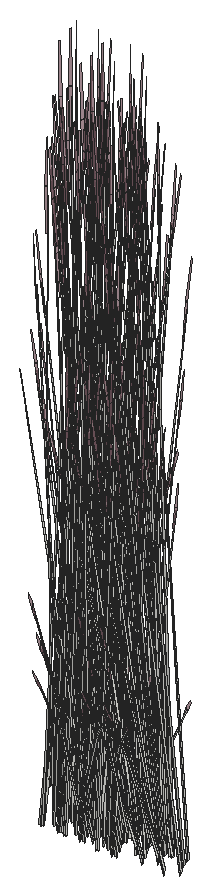
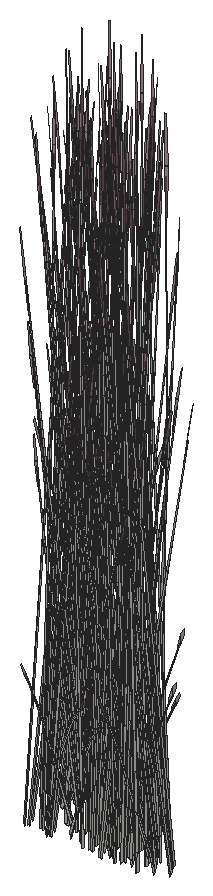
# SketchUp Ruby script. Lengths in inches.
U = 1.inch
M = Sketchup.active_model
def pt(a) = Geom::Point3d.new(a.map { |v| v * U })
def face(e, loops, mat)
  f = e.add_face(loops[0].map { |a| pt(a) })
  loops[1..].each { |l| e.add_face(l.map { |a| pt(a) }).erase! }
  f.material = f.back_material = mat if mat
  f
end
# faces: each face lists its corners as indices into pts; further lists are holes
def faces(e, pts, list, mat = nil) = list.each { |f| face(e, (f[0].is_a?(Array) ? f : [f]).map { |l| l.map { |i| pts[i] } }, mat) }
# xy, xz, yz: faces in a plane at the given z, y or x. An outline is a flat list of corners, or four numbers for a rectangle; further outlines are holes
def ring(l) = l.size == 4 ? [[l[0], l[1]], [l[2], l[1]], [l[2], l[3]], [l[0], l[3]]] : l.each_slice(2).to_a
def flat(e, list, mat, &to3) = list.each { |f| face(e, (f[0].is_a?(Array) ? f : [f]).map { |l| ring(l).map { |u, v| to3.(u, v) } }, mat) }
def xy(e, z, list, mat = nil) = flat(e, list, mat) { |x, y| [x, y, z] }
def xz(e, y, list, mat = nil) = flat(e, list, mat) { |x, z| [x, y, z] }
def yz(e, x, list, mat = nil) = flat(e, list, mat) { |y, z| [x, y, z] }
def lines(e, pts, list) = list.each { |a, b| e.add_line(pt(pts[a]), pt(pts[b])) }
# prism: a flat outline (further loops are holes) pulled along v
def prism(e, loops, v, mat = nil)
  f = face(e, loops, mat); d = Geom::Vector3d.new(v.map { |x| x * U })
  f.pushpull(f.normal.samedirection?(d) ? d.length : -d.length)
end
def box(e, o, s, mat = nil) = prism(e, [[o, [o[0] + s[0], o[1], o[2]], [o[0] + s[0], o[1] + s[1], o[2]], [o[0], o[1] + s[1], o[2]]]], [0, 0, s[2]], mat)
def at(x, y, z, deg = 0) = Geom::Transformation.translation(pt([x, y, z])) * Geom::Transformation.rotation(ORIGIN, Z_AXIS, deg.degrees)
def axes(o, x, y, z) = Geom::Transformation.new([*x, 0, *y, 0, *z, 0, *pt(o).to_a, 1])
def part(name) = M.definitions.add(name)
# library, detail: a bought-in or finely detailed component or shape, given as its bounding box
def library(name, o, s) = part(name).tap { |d| box(d.entities, o, s) }
def detail(e, o, s) = box(e.add_group.entities, o, s)
def put(e, d, t, mat = nil) = e.add_instance(d, t).tap { |i| i.material = mat if mat }
def group(e, t, mat = nil) = e.add_group.tap { |g| g.transformation = t; g.material = mat if mat }.entities
root = M.entities
M.materials.add("LightPink_Translucent").color = [144, 107, 117]
M.materials["LightPink_Translucent"].alpha = 0.75
c1 = part("blade")
p = [[2.15,0.21,22],[0,0.17,0],[0.09,0.45,0],[2.18,0.31,22],[2.29,0.31,22],[0.38,0.45,0],
  [2.48,0.24,33],[2.49,0.24,33],[2.48,0.22,33]]
faces(c1.entities,p,[[0,1,2,3],[4,5,2,3],[6,3,4,7],[8,0,3,6]])
c2 = part("seeds")
p = [[0.3,-0.1,1.38],[-0.01,-0.03,1.59],[-0.01,-0.03,0.03],[0.14,-0.07,-0.07],[0.29,-0.03,3],[0.15,0.01,3.11]]
faces(c2.entities,p,[[0,1,2,3],[1,0,4,5]],"LightPink_Translucent")
c3 = part("blade with seeds")
put(c3.entities,c1,at(0,0,0))
put(c3.entities,c2,axes([2.4,0.25,30.99],[1.5799,-0.05474,1.17369],[-0.12525,1.92788,0.29478],[-0.07173,-0.02425,1.56792]))
put(root,c3,axes([347.7,353.87,622.68],[-0.25628,0.30892,-0.51099],[-0.22444,-0.32634,-0.3958],[-0.13021,-0.047,0.97773]))
put(root,c3,axes([347.29,354.76,619.49],[0.00895,0.0735,1.76342],[-0.18044,0.38382,-0.26939],[-0.12817,-0.01935,0.30037]))
put(root,c3,axes([343.2,353.8,620.02],[0.33032,0.23318,-0.49651],[-0.19744,0.41812,0],[0.07523,0.05311,1.57504]))
put(root,c3,axes([344.44,355.23,620.21],[0.39487,0,0],[0,0.48281,0],[0,0,1.78407]))
put(root,c3,axes([347.34,353.01,622.71],[0.02617,0.04654,1.77383],[-0.12614,0.41836,-0.16761],[-0.12775,0.00303,0.31391]))
put(root,c3,axes([344.0625,354.7,620.72],[-0.21202,-0.39143,0.44739],[0.32115,-0.27564,-0.21531],[0.06861,0.04843,1.43643]))
put(root,c3,axes([344.66,354.73,620.03],[0.24637,-0.29097,-0.30978],[0.24637,0.29097,0.30978],[0,-0.09372,1.38974]))
put(root,c3,axes([343.68,354.79,620.67],[-0.04113,-0.53214,-0.29095],[0.42835,-0.03218,-0.50002],[0.07543,-0.07088,1.59708]))
put(root,c3,axes([345.68,355.49,620.36],[0.44609,0.09826,0.45755],[-0.09078,0.55493,0.17955],[-0.06519,-0.05359,1.58856]))
put(root,c3,axes([343.41,355.48,623.05],[-0.29332,-0.1301,0.35414],[0.08555,-0.37955,-0.4572],[0.11809,-0.0348,0.87481]))
put(root,c3,axes([347.32,354.55,622.73],[0.09971,-0.42522,0.48003],[0.32782,0.1454,0.3958],[-0.12892,0.02555,0.9933]))
put(root,c3,axes([342.72,354.69,620.06],[0.36714,0.07646,-0.62353],[-0.07747,0.47163,-0.16365],[0.10956,0.05715,1.37633]))
put(root,c3,axes([347.84,353.55,623.03],[-0.0189,0.47427,-0.1216],[-0.35781,-0.01296,-0.67495],[-0.13781,-0.03295,1.02557]))
put(root,c3,axes([345.56,355.39,620.72],[-0.17124,0.42022,0.44739],[-0.35581,-0.20224,-0.21531],[0,-0.09687,1.43643]))
put(root,c3,axes([344.28,354.97,620.26],[-0.21881,-0.29821,-0.06488],[0.23965,-0.27324,-0.29416],[0.0679,-0.01924,0.97024]))
put(root,c3,axes([347.29,354.43,622.73],[-0.12963,-0.31798,0.0643],[0.23638,-0.15564,0.50621],[-0.1042,0.03071,0.77189]))
put(root,c3,axes([343.62,353.61,620.03],[0.32928,0.11539,-0.30978],[-0.08291,0.40636,0.30978],[0.06638,-0.04686,1.38974]))
put(root,c3,axes([343.64,354.51,622.73],[0.2423,0.19613,0.0643],[-0.14107,0.2793,0.50621],[0.07768,-0.0903,0.77189]))
put(root,c3,axes([345.4375,356.37,620.47],[0.37926,-0.12378,0.17642],[0.09365,0.46065,0.35086],[-0.03382,-0.06712,1.60407]))
put(root,c3,axes([347.125,354.28,620.77],[0.22533,-0.03337,1.1486],[-0.14293,0.29403,0.84392],[-0.11135,-0.04411,0.25299]))
put(root,c3,axes([343.57,354.43,622.73],[0.08753,0.42921,0.48003],[-0.34336,0.07449,0.3958],[0.1012,-0.10094,0.9933]))
put(root,c3,axes([344.21,354.59,620.62],[0.06809,-0.4162,0.1448],[0.33266,0.07225,-0.41347],[0.06054,0.04274,1.26744]))
put(root,c3,axes([344.68,353.86,620.48],[-0.33032,-0.23318,0.49651],[0.19744,-0.41812,0],[0.07523,0.05311,1.57504]))
put(root,c3,axes([346.56,356.4,620.47],[0.10196,-0.46348,0.17642],[0.3731,0.13116,0.35086],[-0.06445,0.00226,1.60407]))
put(root,c3,axes([346.3,355.4375,620.3],[-0.32829,-0.4014,-0.06131],[0.32849,-0.40164,0],[-0.01146,-0.01402,1.75571]))
put(root,c3,axes([344.39,356.3,620.18],[0.37054,-0.15823,-0.19198],[0.1302,0.45581,0.00008],[0.0409,-0.01749,1.73897]))
put(root,c3,axes([343.67,355.6,622.73],[0.12963,0.31798,0.0643],[-0.23638,0.15564,0.50621],[0.1042,-0.03071,0.77189]))
put(root,c3,axes([343.53,355.61,623.03],[-0.17758,-0.42229,-0.1216],[0.31518,-0.20752,-0.67495],[0.13282,-0.05572,1.02557]))
put(root,c3,axes([343.65,355.49,622.73],[-0.09971,0.42522,0.48003],[-0.32782,-0.1454,0.3958],[0.12892,-0.02555,0.9933]))
put(root,c3,axes([347.56,354.55,623.05],[0.29332,0.1301,0.35414],[-0.08555,0.37955,-0.4572],[-0.11809,0.0348,0.87481]))
put(root,c3,axes([345.64,354.98,620.36],[0.15345,0.52148,0.45755],[-0.43845,0.18134,0.17955],[0.00536,-0.09582,1.58856]))
put(root,c3,axes([346.01,356.26,620.2],[-0.11516,-0.40207,0],[0.32884,-0.1408,0],[0,0,1.54371]))
put(root,c3,axes([348.47,355.43,620.06],[-0.36714,-0.07646,-0.62353],[0.07747,-0.47163,-0.16365],[-0.10956,-0.05715,1.37633]))
put(root,c3,axes([347.89,353.73,623.05],[0.20082,0.29199,0.35414],[-0.2293,0.2764,-0.4572],[-0.1165,-0.04206,0.87481]))
put(root,c3,axes([343.52,355.25,622.68],[0.09562,-0.42421,-0.51099],[0.32782,0.1454,-0.3958],[0.13199,-0.0389,0.97773]))
put(root,c3,axes([344.34,355.52,620.77],[-0.21807,0.07699,1.1486],[0.10265,-0.31819,0.84392],[0.11568,0.02177,0.25299]))
put(root,c3,axes([347.99,356.32,620.02],[-0.33032,-0.23318,-0.49651],[0.19744,-0.41812,0],[-0.07523,-0.05311,1.57504]))
put(root,c3,axes([344.98,354.07,620.03],[0.08291,0.40636,-0.30978],[-0.32928,0.11539,0.30978],[0.06638,0.04686,1.38974]))
put(root,c3,axes([347.15,355.22,620.47],[-0.2773,-0.3397,0.17642],[0.27945,-0.32949,0.35086],[-0.03063,0.06937,1.60407]))
put(root,c3,axes([343.72,355.4375,622.53],[0.29332,0.1301,-0.35414],[-0.08555,0.37955,0.4572],[0.11809,-0.0348,0.87481]))
put(root,c3,axes([346.1875,355.02,620.21],[0,-0.53961,0],[0.44133,0,0],[0,0,1.79456]))
put(root,c3,axes([345.78,355.12,620.43],[0.39767,0.22603,0.24065],[-0.19139,0.46966,0.50002],[0,-0.10827,1.60543]))
put(root,c3,axes([344.17,354.72,620.67],[0.35635,-0.30962,-0.29095],[0.23697,0.43749,-0.50002],[0.08792,0.04443,1.59708]))
put(root,c3,axes([345.65,354.8,620.72],[-0.38326,0.02879,0.44739],[-0.03466,-0.47788,-0.21531],[0.06861,-0.04843,1.43643]))
put(root,c3,axes([345.23,354.67,623.05],[-0.30722,0.06665,0.35414],[-0.08112,-0.381,-0.4572],[0.08804,-0.10234,0.87481]))
put(root,c3,axes([343.87,355.36,619.98],[-0.22732,0.05597,1.41583],[-0.03618,-0.44548,0.08104],[0.15921,-0.06743,0.80566]))
put(root,c3,axes([345.47,353.98,620.47],[-0.10196,0.46348,0.17642],[-0.3731,-0.13116,0.35086],[0.06445,-0.00226,1.60407]))
put(root,c3,axes([344.12,355.07,619.49],[-0.01845,-0.0708,1.76342],[0.12793,-0.41416,-0.26939],[0.12905,-0.00596,0.30037]))
put(root,c3,axes([342.92,354.97,621.875],[-0.14639,0.01056,1.71376],[0.09712,-0.45778,0.13857],[0.20862,0.02831,0.73262]))
put(root,c3,axes([343.27,354.45,619.59],[-0.3474,0.18671,1.28929],[-0.11057,-0.53572,0.50096],[0.21332,0.00891,1.46642]))
put(root,c3,axes([346.6,354.01,620.47],[-0.37926,0.12378,0.17642],[-0.09365,-0.46065,0.35086],[0.03382,0.06712,1.60407]))
put(root,c3,axes([343.45,355.4,622.98],[0.31014,-0.20596,-0.71045],[0.17284,0.42397,0.08574],[0.14985,-0.04816,1.00501]))
put(root,c3,axes([348.88,355.5,620.67],[-0.35635,0.30962,-0.29095],[-0.23697,-0.43749,-0.50002],[-0.08792,-0.04443,1.59708]))
put(root,c3,axes([345.98,354.68,620.36],[-0.29264,0.42323,0.45755],[-0.34767,-0.3736,0.17955],[0.07055,-0.04224,1.58856]))
put(root,c3,axes([344.5,354.95,622.72],[0.04898,-0.07104,1.74944],[-0.06269,-0.43574,-0.27667],[0.12289,-0.08262,0.14031]))
put(root,c3,axes([346.48,355.35,620.21],[0.24637,0.30123,0],[-0.24637,0.30123,0],[0,0,1.69266]))
put(root,c3,axes([344.87,353.62,620.375],[0.22066,-0.46731,0],[0.36918,0.26061,-0.51607],[0.08408,0.05936,1.63711]))
put(root,c3,axes([348.08,356.15,620.03],[-0.08291,-0.40636,-0.30978],[0.32928,-0.11539,0.30978],[-0.06638,-0.04686,1.38974]))
put(root,c3,axes([345.07,353.9,620.02],[0.33032,0.23318,-0.49651],[-0.19744,0.41812,0],[0.07523,0.05311,1.57504]))
put(root,c3,axes([346.36,354.89,620.38],[-0.44609,-0.09826,0.49198],[0.09078,-0.55493,0.19306],[0.06519,0.05359,1.70813]))
put(root,c3,axes([345.28,355.58,623.05],[-0.29332,-0.1301,0.35414],[0.08555,-0.37955,-0.4572],[0.11809,-0.0348,0.87481]))
put(root,c3,axes([347.8,354.68,620.33],[-0.32829,0.39208,0.30756],[-0.32849,-0.38796,-0.36492],[-0.01146,-0.11134,1.64885]))
put(root,c3,axes([346.49,355.14,620.21],[0.39487,0,0],[0,0.48281,0],[0,0,1.78407]))
put(root,c3,axes([346.11,354.61,620.72],[-0.21202,-0.39143,0.44739],[0.32115,-0.27564,-0.21531],[0.06861,0.04843,1.43643]))
put(root,c3,axes([346.15,355.07,620.26],[-0.21881,-0.29821,-0.06488],[0.23965,-0.27324,-0.29416],[0.0679,-0.01924,0.97024]))
put(root,c3,axes([349.28,355.64,620.46],[-0.34464,-0.37536,-0.25192],[0.29,-0.42149,0.5513],[-0.0928,0.04391,1.68216]))
put(root,c3,axes([348.66,355.28,620.21],[-0.21202,-0.39143,-0.44739],[0.32115,-0.27564,0.21531],[-0.06861,-0.04843,1.43643]))
put(root,c3,axes([345.51,354.61,622.73],[0.2423,0.19613,0.0643],[-0.14107,0.2793,0.50621],[0.07768,-0.0903,0.77189]))
put(root,c3,axes([345.67,353.52,620.03],[0.32928,0.11539,-0.30978],[-0.08291,0.40636,0.30978],[0.06638,-0.04686,1.38974]))
put(root,c3,axes([345.44,354.53,622.73],[0.08753,0.42921,0.48003],[-0.34336,0.07449,0.3958],[0.1012,-0.10094,0.9933]))
put(root,c3,axes([348.38,356.36,620.48],[0.33032,0.23318,0.49651],[-0.19744,0.41812,0],[-0.07523,-0.05311,1.57504]))
put(root,c3,axes([348.6875,355.5,620.4375],[0.09355,-0.55261,-0.23429],[0.44354,0.09633,0.51271],[-0.0775,-0.07631,1.5644]))
put(root,c3,axes([346.25,354.5,620.62],[0.06809,-0.4162,0.1448],[0.33266,0.07225,-0.41347],[0.06054,0.04274,1.26744]))
put(root,c3,axes([345.55,355.7,622.73],[0.12963,0.31798,0.0643],[-0.23638,0.15564,0.50621],[0.1042,-0.03071,0.77189]))
put(root,c3,axes([348.85,355.63,620.62],[-0.06809,0.4162,0.1448],[-0.33266,-0.07225,-0.41347],[-0.06054,-0.04274,1.26744]))
put(root,c3,axes([345.4,355.71,623.03],[-0.17758,-0.42229,-0.1216],[0.31518,-0.20752,-0.67495],[0.13282,-0.05572,1.02557]))
put(root,c3,axes([345.52,355.59,622.73],[-0.09971,0.42522,0.48003],[-0.32782,-0.1454,0.3958],[0.12892,-0.02555,0.9933]))
put(root,c3,axes([347.73,354.9,620.48],[0,0.46636,0.49651],[-0.39487,0,0],[0,-0.10622,1.57504]))
put(root,c3,axes([346.72,353.77,620.48],[-0.33032,-0.23318,0.49651],[0.19744,-0.41812,0],[0.07523,0.05311,1.57504]))
put(root,c3,axes([346.4375,356.21,620.18],[0.37054,-0.15823,-0.19198],[0.1302,0.45581,0.00008],[0.0409,-0.01749,1.73897]))
put(root,c3,axes([345.39,355.35,622.68],[0.09562,-0.42421,-0.51099],[0.32782,0.1454,-0.3958],[0.13199,-0.0389,0.97773]))
put(root,c3,axes([345.59,355.54,622.53],[0.29332,0.1301,-0.35414],[-0.08555,0.37955,0.4572],[0.11809,-0.0348,0.87481]))
put(root,c3,axes([348.74,355.24,620.36],[0.44609,0.09826,0.45755],[-0.09078,0.55493,0.17955],[-0.06519,-0.05359,1.58856]))
put(root,c3,axes([347.02,353.98,620.03],[0.08291,0.40636,-0.30978],[-0.32928,0.11539,0.30978],[0.06638,0.04686,1.38974]))
put(root,c3,axes([345.74,355.47,619.98],[-0.22732,0.05597,1.41583],[-0.03618,-0.44548,0.08104],[0.15921,-0.06743,0.80566]))
put(root,c3,axes([348.625,355.14,620.72],[-0.17124,0.42022,0.44739],[-0.35581,-0.20224,-0.21531],[0,-0.09687,1.43643]))
put(root,c3,axes([345.99,355.17,619.49],[-0.01845,-0.0708,1.76342],[0.12793,-0.41416,-0.26939],[0.12905,-0.00596,0.30037]))
put(root,c3,axes([346.22,354.63,620.67],[0.35635,-0.30962,-0.29095],[0.23697,0.43749,-0.50002],[0.08792,0.04443,1.59708]))
put(root,c3,axes([344.79,355.07,621.875],[-0.14639,0.01056,1.71376],[0.09712,-0.45778,0.13857],[0.20862,0.02831,0.73262]))
put(root,c3,axes([351.97,353.97,621.875],[0.14639,-0.01056,1.71376],[-0.09712,0.45778,0.13857],[-0.20862,-0.02831,0.73262]))
put(root,c3,axes([347.28,354.58,623.05],[-0.30722,0.06665,0.35414],[-0.08112,-0.381,-0.4572],[0.08804,-0.10234,0.87481]))
put(root,c3,axes([348.5,356.12,620.47],[0.37926,-0.12378,0.17642],[0.09365,0.46065,0.35086],[-0.03382,-0.06712,1.60407]))
put(root,c3,axes([348.99,356.2,620.2],[-0.35581,-0.20937,0],[0.17124,-0.43505,0],[0,0,1.62707]))
put(root,c3,axes([345.33,355.5,622.98],[0.31014,-0.20596,-0.71045],[0.17284,0.42397,0.08574],[0.14985,-0.04816,1.00501]))
put(root,c3,axes([346.37,355.05,622.72],[0.04898,-0.07104,1.74944],[-0.06269,-0.43574,-0.27667],[0.12289,-0.08262,0.14031]))
put(root,c3,axes([345.32,354.36,619.59],[-0.3474,0.18671,1.28929],[-0.11057,-0.53572,0.50096],[0.21332,0.00891,1.46642]))
put(root,c3,axes([349.63,356.15,620.47],[0.10196,-0.46348,0.17642],[0.3731,0.13116,0.35086],[-0.06445,0.00226,1.60407]))
put(root,c3,axes([349.36,355.1875,620.3],[-0.32829,-0.4014,-0.06131],[0.32849,-0.40164,0],[-0.01146,-0.01402,1.75571]))
put(root,c3,axes([346.91,353.53,620.375],[0.22066,-0.46731,0],[0.36918,0.26061,-0.51607],[0.08408,0.05936,1.63711]))
put(root,c3,axes([347.12,353.81,620.02],[0.33032,0.23318,-0.49651],[-0.19744,0.41812,0],[0.07523,0.05311,1.57504]))
put(root,c3,axes([348.7,354.72,620.36],[0.15345,0.52148,0.45755],[-0.43845,0.18134,0.17955],[0.00536,-0.09582,1.58856]))
put(root,c3,axes([352.74,354.3,621.34],[0.10032,-0.06746,1.77064],[0.0346,0.47103,0.13857],[-0.2173,0.0625,0.63284]))
put(root,c3,axes([349.07,356.01,620.2],[-0.11516,-0.40207,0],[0.32884,-0.1408,0],[0,0,1.54371]))
put(root,c3,axes([347.32,355.49,623.05],[-0.29332,-0.1301,0.35414],[0.08555,-0.37955,-0.4572],[0.11809,-0.0348,0.87481]))
put(root,c3,axes([346.63,354.7,620.06],[0.36714,0.07646,-0.62353],[-0.07747,0.47163,-0.16365],[0.10956,0.05715,1.37633]))
put(root,c3,axes([348.2,354.98,620.26],[-0.21881,-0.29821,-0.06488],[0.23965,-0.27324,-0.29416],[0.0679,-0.01924,0.97024]))
put(root,c3,axes([351.66,354.61,622.72],[-0.05763,0.06055,1.74944],[0.0049,0.44239,-0.27667],[-0.13211,0.05753,0.14031]))
put(root,c3,axes([347.55,354.52,622.73],[0.2423,0.19613,0.0643],[-0.14107,0.2793,0.50621],[0.07768,-0.0903,0.77189]))
put(root,c3,axes([351.84,354.36,622.53],[-0.29332,-0.1301,-0.35414],[0.08555,-0.37955,0.4572],[-0.11809,0.0348,0.87481]))
put(root,c3,axes([350.21,354.97,620.47],[-0.2773,-0.3397,0.17642],[0.27945,-0.32949,0.35086],[-0.03063,0.06937,1.60407]))
put(root,c3,axes([349.25,354.77,620.21],[0,-0.53961,0],[0.44133,0,0],[0,0,1.79456]))
put(root,c3,axes([347.49,354.4375,622.73],[0.08753,0.42921,0.48003],[-0.34336,0.07449,0.3958],[0.1012,-0.10094,0.9933]))
put(root,c3,axes([348.84,354.87,620.43],[0.39767,0.22603,0.24065],[-0.19139,0.46966,0.50002],[0,-0.10827,1.60543]))
put(root,c3,axes([348.72,354.55,620.72],[-0.38326,0.02879,0.44739],[-0.03466,-0.47788,-0.21531],[0.06861,-0.04843,1.43643]))
put(root,c3,axes([352.05,354.55,622.68],[-0.09562,0.42421,-0.51099],[-0.32782,-0.1454,-0.3958],[-0.13199,0.0389,0.97773]))
put(root,c3,axes([348.54,353.73,620.47],[-0.10196,0.46348,0.17642],[-0.3731,-0.13116,0.35086],[0.06445,-0.00226,1.60407]))
put(root,c3,axes([352.29,353.64,622.68],[-0.25628,0.30892,-0.51099],[-0.22444,-0.32634,-0.3958],[-0.13021,-0.047,0.97773]))
put(root,c3,axes([351.88,354.53,619.49],[0.00895,0.0735,1.76342],[-0.18044,0.38382,-0.26939],[-0.12817,-0.01935,0.30037]))
put(root,c3,axes([347.59,355.61,622.73],[0.12963,0.31798,0.0643],[-0.23638,0.15564,0.50621],[0.1042,-0.03071,0.77189]))
put(root,c3,axes([351.93,352.77,622.71],[0.02617,0.04654,1.77383],[-0.12614,0.41836,-0.16761],[-0.12775,0.00303,0.31391]))
put(root,c3,axes([347.45,355.62,623.03],[-0.17758,-0.42229,-0.1216],[0.31518,-0.20752,-0.67495],[0.13282,-0.05572,1.02557]))
put(root,c3,axes([347.57,355.5,622.73],[-0.09971,0.42522,0.48003],[-0.32782,-0.1454,0.3958],[0.12892,-0.02555,0.9933]))
put(root,c3,axes([349.67,353.76,620.47],[-0.37926,0.12378,0.17642],[-0.09365,-0.46065,0.35086],[0.03382,0.06712,1.60407]))
put(root,c3,axes([351.91,354.3125,622.73],[0.09971,-0.42522,0.48003],[0.32782,0.1454,0.3958],[-0.12892,0.02555,0.9933]))
put(root,c3,axes([352.03,354.19,623.03],[0.17758,0.42229,-0.1216],[-0.31518,0.20752,-0.67495],[-0.13282,0.05572,1.02557]))
put(root,c3,axes([349.05,354.43,620.36],[-0.29264,0.42323,0.45755],[-0.34767,-0.3736,0.17955],[0.07055,-0.04224,1.58856]))
put(root,c3,axes([352.43,353.3125,623.03],[-0.0189,0.47427,-0.1216],[-0.35781,-0.01296,-0.67495],[-0.13781,-0.03295,1.02557]))
put(root,c3,axes([349.54,355.1,620.21],[0.24637,0.30123,0],[-0.24637,0.30123,0],[0,0,1.69266]))
put(root,c3,axes([349.54,354.74,620.72],[0.17124,-0.42022,0.44739],[0.35581,0.20224,-0.21531],[0,0.09687,1.43643]))
put(root,c3,axes([351.89,354.2,622.73],[-0.12963,-0.31798,0.0643],[0.23638,-0.15564,0.50621],[-0.1042,0.03071,0.77189]))
put(root,c3,axes([349.43,354.64,620.38],[-0.44609,-0.09826,0.49198],[0.09078,-0.55493,0.19306],[0.06519,0.05359,1.70813]))
put(root,c3,axes([351.72,354.05,620.77],[0.22533,-0.03337,1.1486],[-0.14293,0.29403,0.84392],[-0.11135,-0.04411,0.25299]))
put(root,c3,axes([347.43,355.26,622.68],[0.09562,-0.42421,-0.51099],[0.32782,0.1454,-0.3958],[0.13199,-0.0389,0.97773]))
put(root,c3,axes([349.55,354.89,620.21],[0.39487,0,0],[0,0.48281,0],[0,0,1.78407]))
put(root,c3,axes([349.17,354.36,620.72],[-0.21202,-0.39143,0.44739],[0.32115,-0.27564,-0.21531],[0.06861,0.04843,1.43643]))
put(root,c3,axes([347.63,355.45,622.53],[0.29332,0.1301,-0.35414],[-0.08555,0.37955,0.4572],[0.11809,-0.0348,0.87481]))
put(root,c3,axes([347.78,355.375,619.98],[-0.22732,0.05597,1.41583],[-0.03618,-0.44548,0.08104],[0.15921,-0.06743,0.80566]))
put(root,c3,axes([348.03,355.08,619.49],[-0.01845,-0.0708,1.76342],[0.12793,-0.41416,-0.26939],[0.12905,-0.00596,0.30037]))
put(root,c3,axes([348.73,353.27,620.03],[0.32928,0.11539,-0.30978],[-0.08291,0.40636,0.30978],[0.06638,-0.04686,1.38974]))
put(root,c3,axes([352.15,354.32,623.05],[0.29332,0.1301,0.35414],[-0.08555,0.37955,-0.4572],[-0.11809,0.0348,0.87481]))
put(root,c3,axes([346.83,354.98,621.875],[-0.14639,0.01056,1.71376],[0.09712,-0.45778,0.13857],[0.20862,0.02831,0.73262]))
put(root,c3,axes([354.13,353.69,621.875],[0.14639,-0.01056,1.71376],[-0.09712,0.45778,0.13857],[-0.20862,-0.02831,0.73262]))
put(root,c3,axes([353.0625,355.19,620.06],[-0.36714,-0.07646,-0.62353],[0.07747,-0.47163,-0.16365],[-0.10956,-0.05715,1.37633]))
put(root,c3,axes([347.37,355.41,622.98],[0.31014,-0.20596,-0.71045],[0.17284,0.42397,0.08574],[0.14985,-0.04816,1.00501]))
put(root,c3,axes([349.32,354.25,620.62],[0.06809,-0.4162,0.1448],[0.33266,0.07225,-0.41347],[0.06054,0.04274,1.26744]))
put(root,c3,axes([352.48,353.5,623.05],[0.20082,0.29199,0.35414],[-0.2293,0.2764,-0.4572],[-0.1165,-0.04206,0.87481]))
put(root,c3,axes([348.41,354.96,622.72],[0.04898,-0.07104,1.74944],[-0.06269,-0.43574,-0.27667],[0.12289,-0.08262,0.14031]))
put(root,c3,axes([349.79,353.52,620.48],[-0.33032,-0.23318,0.49651],[0.19744,-0.41812,0],[0.07523,0.05311,1.57504]))
put(root,c3,axes([352.58,356.09,620.02],[-0.33032,-0.23318,-0.49651],[0.19744,-0.41812,0],[-0.07523,-0.05311,1.57504]))
put(root,c3,axes([349.5,355.96,620.18],[0.37054,-0.15823,-0.19198],[0.1302,0.45581,0.00008],[0.0409,-0.01749,1.73897]))
put(root,c3,axes([352.78,356.37,620.375],[-0.22066,0.46731,0],[-0.36918,-0.26061,-0.51607],[-0.08408,-0.05936,1.63711]))
put(root,c3,axes([354.89,354.02,621.34],[0.10032,-0.06746,1.77064],[0.0346,0.47103,0.13857],[-0.2173,0.0625,0.63284]))
put(root,c3,axes([353.48,355.26,620.67],[-0.35635,0.30962,-0.29095],[-0.23697,-0.43749,-0.50002],[-0.08792,-0.04443,1.59708]))
put(root,c3,axes([353.82,354.34,622.72],[-0.05763,0.06055,1.74944],[0.0049,0.44239,-0.27667],[-0.13211,0.05753,0.14031]))
put(root,c3,axes([350.09,353.73,620.03],[0.08291,0.40636,-0.30978],[-0.32928,0.11539,0.30978],[0.06638,0.04686,1.38974]))
put(root,c3,axes([352.67,355.91,620.03],[-0.08291,-0.40636,-0.30978],[0.32928,-0.11539,0.30978],[-0.06638,-0.04686,1.38974]))
put(root,c3,axes([349.28,354.38,620.67],[0.35635,-0.30962,-0.29095],[0.23697,0.43749,-0.50002],[0.08792,0.04443,1.59708]))
put(root,c3,axes([354,354.09,622.53],[-0.29332,-0.1301,-0.35414],[0.08555,-0.37955,0.4572],[-0.11809,0.0348,0.87481]))
put(root,c3,axes([354.2,354.28,622.68],[-0.09562,0.42421,-0.51099],[-0.32782,-0.1454,-0.3958],[-0.13199,0.0389,0.97773]))
put(root,c3,axes([352.39,354.45,620.33],[-0.32829,0.39208,0.30756],[-0.32849,-0.38796,-0.36492],[-0.01146,-0.11134,1.64885]))
put(root,c3,axes([354.45,353.36,622.68],[-0.25628,0.30892,-0.51099],[-0.22444,-0.32634,-0.3958],[-0.13021,-0.047,0.97773]))
put(root,c3,axes([354.04,354.25,619.49],[0.00895,0.0735,1.76342],[-0.18044,0.38382,-0.26939],[-0.12817,-0.01935,0.30037]))
put(root,c3,axes([348.38,354.11,619.59],[-0.3474,0.18671,1.28929],[-0.11057,-0.53572,0.50096],[0.21332,0.00891,1.46642]))
put(root,c3,axes([353.88,355.4,620.46],[-0.34464,-0.37536,-0.25192],[0.29,-0.42149,0.5513],[-0.0928,0.04391,1.68216]))
put(root,c3,axes([353.25,355.04,620.21],[-0.21202,-0.39143,-0.44739],[0.32115,-0.27564,0.21531],[-0.06861,-0.04843,1.43643]))
put(root,c3,axes([354.09,352.5,622.71],[0.02617,0.04654,1.77383],[-0.12614,0.41836,-0.16761],[-0.12775,0.00303,0.31391]))
put(root,c3,axes([349.98,353.28,620.375],[0.22066,-0.46731,0],[0.36918,0.26061,-0.51607],[0.08408,0.05936,1.63711]))
put(root,c3,axes([354.07,354.04,622.73],[0.09971,-0.42522,0.48003],[0.32782,0.1454,0.3958],[-0.12892,0.02555,0.9933]))
put(root,c3,axes([354.1875,353.92,623.03],[0.17758,0.42229,-0.1216],[-0.31518,0.20752,-0.67495],[-0.13282,0.05572,1.02557]))
put(root,c3,axes([350.18,353.56,620.02],[0.33032,0.23318,-0.49651],[-0.19744,0.41812,0],[0.07523,0.05311,1.57504]))
put(root,c3,axes([354.59,353.04,623.03],[-0.0189,0.47427,-0.1216],[-0.35781,-0.01296,-0.67495],[-0.13781,-0.03295,1.02557]))
put(root,c3,axes([354.04,353.93,622.73],[-0.12963,-0.31798,0.0643],[0.23638,-0.15564,0.50621],[-0.1042,0.03071,0.77189]))
put(root,c3,axes([352.97,356.125,620.48],[0.33032,0.23318,0.49651],[-0.19744,0.41812,0],[-0.07523,-0.05311,1.57504]))
put(root,c3,axes([353.28,355.27,620.4375],[0.09355,-0.55261,-0.23429],[0.44354,0.09633,0.51271],[-0.0775,-0.07631,1.5644]))
put(root,c3,axes([350.39,355.24,623.05],[-0.29332,-0.1301,0.35414],[0.08555,-0.37955,-0.4572],[0.11809,-0.0348,0.87481]))
put(root,c3,axes([353.875,353.77,620.77],[0.22533,-0.03337,1.1486],[-0.14293,0.29403,0.84392],[-0.11135,-0.04411,0.25299]))
put(root,c3,axes([353.44,355.4,620.62],[-0.06809,0.4162,0.1448],[-0.33266,-0.07225,-0.41347],[-0.06054,-0.04274,1.26744]))
put(root,c3,axes([349.7,354.45,620.06],[0.36714,0.07646,-0.62353],[-0.07747,0.47163,-0.16365],[0.10956,0.05715,1.37633]))
put(root,c3,axes([351.26,354.73,620.26],[-0.21881,-0.29821,-0.06488],[0.23965,-0.27324,-0.29416],[0.0679,-0.01924,0.97024]))
put(root,c3,axes([352.32,354.67,620.48],[0,0.46636,0.49651],[-0.39487,0,0],[0,-0.10622,1.57504]))
put(root,c3,axes([350.62,354.27,622.73],[0.2423,0.19613,0.0643],[-0.14107,0.2793,0.50621],[0.07768,-0.0903,0.77189]))
put(root,c3,axes([350.55,354.1875,622.73],[0.08753,0.42921,0.48003],[-0.34336,0.07449,0.3958],[0.1012,-0.10094,0.9933]))
put(root,c3,axes([354.31,354.04,623.05],[0.29332,0.1301,0.35414],[-0.08555,0.37955,-0.4572],[-0.11809,0.0348,0.87481]))
put(root,c3,axes([350.66,355.36,622.73],[0.12963,0.31798,0.0643],[-0.23638,0.15564,0.50621],[0.1042,-0.03071,0.77189]))
put(root,c3,axes([355.22,354.92,620.06],[-0.36714,-0.07646,-0.62353],[0.07747,-0.47163,-0.16365],[-0.10956,-0.05715,1.37633]))
put(root,c3,axes([350.51,355.37,623.03],[-0.17758,-0.42229,-0.1216],[0.31518,-0.20752,-0.67495],[0.13282,-0.05572,1.02557]))
put(root,c3,axes([350.63,355.25,622.73],[-0.09971,0.42522,0.48003],[-0.32782,-0.1454,0.3958],[0.12892,-0.02555,0.9933]))
put(root,c3,axes([354.64,353.23,623.05],[0.20082,0.29199,0.35414],[-0.2293,0.2764,-0.4572],[-0.1165,-0.04206,0.87481]))
put(root,c3,axes([353.33,355,620.36],[0.44609,0.09826,0.45755],[-0.09078,0.55493,0.17955],[-0.06519,-0.05359,1.58856]))
put(root,c3,axes([353.22,354.9,620.72],[-0.17124,0.42022,0.44739],[-0.35581,-0.20224,-0.21531],[0,-0.09687,1.43643]))
put(root,c3,axes([354.74,355.8125,620.02],[-0.33032,-0.23318,-0.49651],[0.19744,-0.41812,0],[-0.07523,-0.05311,1.57504]))
put(root,c3,axes([354.9375,356.09,620.375],[-0.22066,0.46731,0],[-0.36918,-0.26061,-0.51607],[-0.08408,-0.05936,1.63711]))
put(root,c3,axes([353.09,355.89,620.47],[0.37926,-0.12378,0.17642],[0.09365,0.46065,0.35086],[-0.03382,-0.06712,1.60407]))
put(root,c3,axes([350.5,355.01,622.68],[0.09562,-0.42421,-0.51099],[0.32782,0.1454,-0.3958],[0.13199,-0.0389,0.97773]))
put(root,c3,axes([353.58,355.96,620.2],[-0.35581,-0.20937,0],[0.17124,-0.43505,0],[0,0,1.62707]))
put(root,c3,axes([351.32,355.28,620.77],[-0.21807,0.07699,1.1486],[0.10265,-0.31819,0.84392],[0.11568,0.02177,0.25299]))
